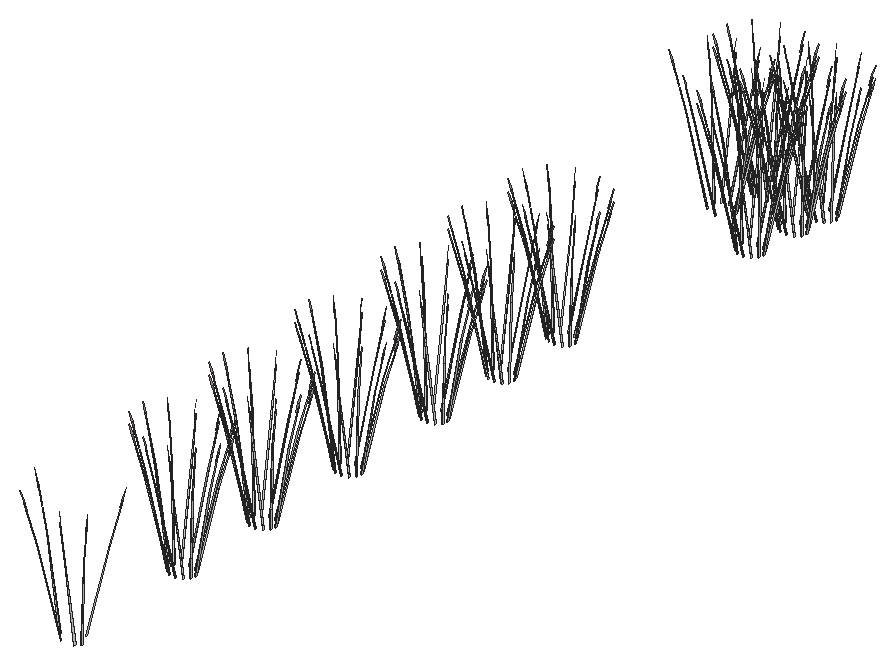
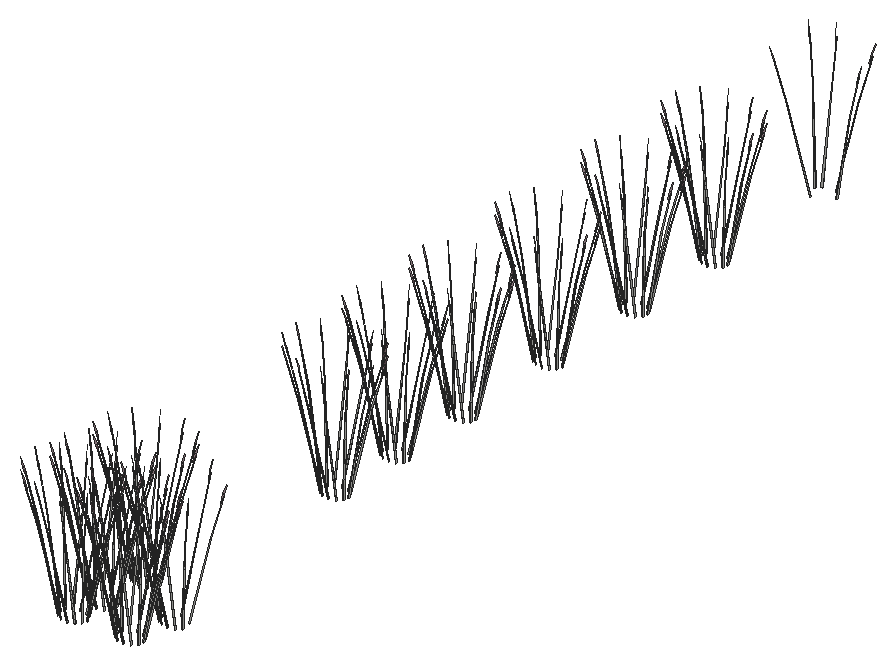
# SketchUp Ruby script. Lengths in inches.
U = 1.inch
M = Sketchup.active_model
def pt(a) = Geom::Point3d.new(a.map { |v| v * U })
def face(e, loops, mat)
  f = e.add_face(loops[0].map { |a| pt(a) })
  loops[1..].each { |l| e.add_face(l.map { |a| pt(a) }).erase! }
  f.material = f.back_material = mat if mat
  f
end
# faces: each face lists its corners as indices into pts; further lists are holes
def faces(e, pts, list, mat = nil) = list.each { |f| face(e, (f[0].is_a?(Array) ? f : [f]).map { |l| l.map { |i| pts[i] } }, mat) }
# xy, xz, yz: faces in a plane at the given z, y or x. An outline is a flat list of corners, or four numbers for a rectangle; further outlines are holes
def ring(l) = l.size == 4 ? [[l[0], l[1]], [l[2], l[1]], [l[2], l[3]], [l[0], l[3]]] : l.each_slice(2).to_a
def flat(e, list, mat, &to3) = list.each { |f| face(e, (f[0].is_a?(Array) ? f : [f]).map { |l| ring(l).map { |u, v| to3.(u, v) } }, mat) }
def xy(e, z, list, mat = nil) = flat(e, list, mat) { |x, y| [x, y, z] }
def xz(e, y, list, mat = nil) = flat(e, list, mat) { |x, z| [x, y, z] }
def yz(e, x, list, mat = nil) = flat(e, list, mat) { |y, z| [x, y, z] }
def lines(e, pts, list) = list.each { |a, b| e.add_line(pt(pts[a]), pt(pts[b])) }
# prism: a flat outline (further loops are holes) pulled along v
def prism(e, loops, v, mat = nil)
  f = face(e, loops, mat); d = Geom::Vector3d.new(v.map { |x| x * U })
  f.pushpull(f.normal.samedirection?(d) ? d.length : -d.length)
end
def box(e, o, s, mat = nil) = prism(e, [[o, [o[0] + s[0], o[1], o[2]], [o[0] + s[0], o[1] + s[1], o[2]], [o[0], o[1] + s[1], o[2]]]], [0, 0, s[2]], mat)
def at(x, y, z, deg = 0) = Geom::Transformation.translation(pt([x, y, z])) * Geom::Transformation.rotation(ORIGIN, Z_AXIS, deg.degrees)
def axes(o, x, y, z) = Geom::Transformation.new([*x, 0, *y, 0, *z, 0, *pt(o).to_a, 1])
def part(name) = M.definitions.add(name)
# library, detail: a bought-in or finely detailed component or shape, given as its bounding box
def library(name, o, s) = part(name).tap { |d| box(d.entities, o, s) }
def detail(e, o, s) = box(e.add_group.entities, o, s)
def put(e, d, t, mat = nil) = e.add_instance(d, t).tap { |i| i.material = mat if mat }
def group(e, t, mat = nil) = e.add_group.tap { |g| g.transformation = t; g.material = mat if mat }.entities
root = M.entities
M.materials.add("LightPink_Translucent").color = [144, 107, 117]
M.materials["LightPink_Translucent"].alpha = 0.75
c1 = part("blade")
p = [[2.15,0.21,22],[0,0.17,0],[0.09,0.45,0],[2.18,0.31,22],[2.29,0.31,22],[0.38,0.45,0],
  [2.48,0.24,33],[2.49,0.24,33],[2.48,0.22,33]]
faces(c1.entities,p,[[0,1,2,3],[4,5,2,3],[6,3,4,7],[8,0,3,6]])
c2 = part("seeds")
p = [[0.3,-0.1,1.38],[-0.01,-0.03,1.59],[-0.01,-0.03,0.03],[0.14,-0.07,-0.07],[0.29,-0.03,3],[0.15,0.01,3.11]]
faces(c2.entities,p,[[0,1,2,3],[1,0,4,5]],"LightPink_Translucent")
c3 = part("blade with seeds")
put(c3.entities,c1,at(0,0,0))
put(c3.entities,c2,axes([2.4,0.25,30.99],[1.5799,-0.05474,1.17369],[-0.12525,1.92788,0.29478],[-0.07173,-0.02425,1.56792]))
put(root,c3,axes([672.56,170.6875,514.19],[-0.10048,-0.4599,0.29394],[0.5744,-0.12144,-0.37948],[0.15428,0.13179,0.72609]))
put(root,c3,axes([674.22,167.95,514.19],[-0.56631,0.0816,0.29394],[-0.14954,-0.46647,-0.37948],[0.16229,-0.12529,0.72609]))
put(root,c3,axes([669.09,168.22,514.19],[0.54068,0.15928,0.29394],[-0.1577,0.46469,-0.37948],[-0.21769,0.04261,0.72609]))
put(root,c3,axes([673.45,167.02,514.19],[-0.4402,0.30062,0.29394],[-0.41671,-0.34326,-0.37948],[0.0634,-0.1744,0.72609]))
put(root,c3,axes([670.85,166.6,514.19],[0.10048,0.4599,0.29394],[-0.5744,0.12144,-0.37948],[-0.15428,-0.13179,0.72609]))
put(root,c3,axes([671.18,198.22,514.19],[0.19614,-0.43908,0.29394],[0.57222,0.12807,-0.37948],[0.05247,0.17678,0.72609]))
put(root,c3,axes([672.22,193.98,514.19],[-0.19614,0.43908,0.29394],[-0.57222,-0.12807,-0.37948],[-0.05247,-0.17678,0.72609]))
put(root,c3,axes([673.7,197.52,514.19],[-0.37017,-0.35748,0.29394],[0.42268,-0.3384,-0.37948],[0.21476,0.05149,0.72609]))
put(root,c3,axes([674.31,196.52,514.19],[-0.54068,-0.15928,0.29394],[0.1577,-0.46469,-0.37948],[0.21769,-0.04261,0.72609]))
put(root,c3,axes([669.7,194.67,514.19],[0.37017,0.35748,0.29394],[-0.42268,0.3384,-0.37948],[-0.21476,-0.05149,0.72609]))
put(root,c3,axes([669.95,197.72,514.19],[0.4402,-0.30062,0.29394],[0.41671,0.34326,-0.37948],[-0.0634,0.1744,0.72609]))
put(root,c3,axes([669.18,196.79,514.19],[0.56631,-0.0816,0.29394],[0.14954,0.46647,-0.37948],[-0.16229,0.12529,0.72609]))
put(root,c3,axes([672.56,198.14,514.19],[-0.10048,-0.4599,0.29394],[0.5744,-0.12144,-0.37948],[0.15428,0.13179,0.72609]))
put(root,c3,axes([674.22,195.4,514.19],[-0.56631,0.0816,0.29394],[-0.14954,-0.46647,-0.37948],[0.16229,-0.12529,0.72609]))
put(root,c3,axes([669.09,195.68,514.19],[0.54068,0.15928,0.29394],[-0.1577,0.46469,-0.37948],[-0.21769,0.04261,0.72609]))
put(root,c3,axes([673.45,194.48,514.19],[-0.4402,0.30062,0.29394],[-0.41671,-0.34326,-0.37948],[0.0634,-0.1744,0.72609]))
put(root,c3,axes([670.85,194.05,514.19],[0.10048,0.4599,0.29394],[-0.5744,0.12144,-0.37948],[-0.15428,-0.13179,0.72609]))
put(root,c3,axes([671.18,218.51,514.19],[0.19614,-0.43908,0.29394],[0.57222,0.12807,-0.37948],[0.05247,0.17678,0.72609]))
put(root,c3,axes([672.22,214.27,514.19],[-0.19614,0.43908,0.29394],[-0.57222,-0.12807,-0.37948],[-0.05247,-0.17678,0.72609]))
put(root,c3,axes([673.7,217.81,514.19],[-0.37017,-0.35748,0.29394],[0.42268,-0.3384,-0.37948],[0.21476,0.05149,0.72609]))
put(root,c3,axes([674.31,216.8125,514.19],[-0.54068,-0.15928,0.29394],[0.1577,-0.46469,-0.37948],[0.21769,-0.04261,0.72609]))
put(root,c3,axes([669.7,214.97,514.19],[0.37017,0.35748,0.29394],[-0.42268,0.3384,-0.37948],[-0.21476,-0.05149,0.72609]))
put(root,c3,axes([669.95,218.01,514.19],[0.4402,-0.30062,0.29394],[0.41671,0.34326,-0.37948],[-0.0634,0.1744,0.72609]))
put(root,c3,axes([669.18,217.08,514.19],[0.56631,-0.0816,0.29394],[0.14954,0.46647,-0.37948],[-0.16229,0.12529,0.72609]))
put(root,c3,axes([672.56,218.4375,514.19],[-0.10048,-0.4599,0.29394],[0.5744,-0.12144,-0.37948],[0.15428,0.13179,0.72609]))
put(root,c3,axes([674.22,215.7,514.19],[-0.56631,0.0816,0.29394],[-0.14954,-0.46647,-0.37948],[0.16229,-0.12529,0.72609]))
put(root,c3,axes([669.09,215.97,514.19],[0.54068,0.15928,0.29394],[-0.1577,0.46469,-0.37948],[-0.21769,0.04261,0.72609]))
put(root,c3,axes([673.45,214.77,514.19],[-0.4402,0.30062,0.29394],[-0.41671,-0.34326,-0.37948],[0.0634,-0.1744,0.72609]))
put(root,c3,axes([670.85,214.35,514.19],[0.10048,0.4599,0.29394],[-0.5744,0.12144,-0.37948],[-0.15428,-0.13179,0.72609]))
put(root,c3,axes([671.18,240.21,514.19],[0.19614,-0.43908,0.29394],[0.57222,0.12807,-0.37948],[0.05247,0.17678,0.72609]))
put(root,c3,axes([672.22,235.97,514.19],[-0.19614,0.43908,0.29394],[-0.57222,-0.12807,-0.37948],[-0.05247,-0.17678,0.72609]))
put(root,c3,axes([673.7,239.51,514.19],[-0.37017,-0.35748,0.29394],[0.42268,-0.3384,-0.37948],[0.21476,0.05149,0.72609]))
put(root,c3,axes([674.31,238.51,514.19],[-0.54068,-0.15928,0.29394],[0.1577,-0.46469,-0.37948],[0.21769,-0.04261,0.72609]))
put(root,c3,axes([669.7,236.66,514.19],[0.37017,0.35748,0.29394],[-0.42268,0.3384,-0.37948],[-0.21476,-0.05149,0.72609]))
put(root,c3,axes([669.95,239.71,514.19],[0.4402,-0.30062,0.29394],[0.41671,0.34326,-0.37948],[-0.0634,0.1744,0.72609]))
put(root,c3,axes([669.18,238.78,514.19],[0.56631,-0.0816,0.29394],[0.14954,0.46647,-0.37948],[-0.16229,0.12529,0.72609]))
put(root,c3,axes([672.56,240.13,514.19],[-0.10048,-0.4599,0.29394],[0.5744,-0.12144,-0.37948],[0.15428,0.13179,0.72609]))
put(root,c3,axes([674.22,237.39,514.19],[-0.56631,0.0816,0.29394],[-0.14954,-0.46647,-0.37948],[0.16229,-0.12529,0.72609]))
put(root,c3,axes([669.09,237.67,514.19],[0.54068,0.15928,0.29394],[-0.1577,0.46469,-0.37948],[-0.21769,0.04261,0.72609]))
put(root,c3,axes([673.45,236.46,514.19],[-0.4402,0.30062,0.29394],[-0.41671,-0.34326,-0.37948],[0.0634,-0.1744,0.72609]))
put(root,c3,axes([670.85,236.04,514.19],[0.10048,0.4599,0.29394],[-0.5744,0.12144,-0.37948],[-0.15428,-0.13179,0.72609]))
put(root,c3,axes([671.18,262.05,514.19],[0.19614,-0.43908,0.29394],[0.57222,0.12807,-0.37948],[0.05247,0.17678,0.72609]))
put(root,c3,axes([672.22,257.82,514.19],[-0.19614,0.43908,0.29394],[-0.57222,-0.12807,-0.37948],[-0.05247,-0.17678,0.72609]))
put(root,c3,axes([673.7,261.36,514.19],[-0.37017,-0.35748,0.29394],[0.42268,-0.3384,-0.37948],[0.21476,0.05149,0.72609]))
put(root,c3,axes([674.31,260.35,514.19],[-0.54068,-0.15928,0.29394],[0.1577,-0.46469,-0.37948],[0.21769,-0.04261,0.72609]))
put(root,c3,axes([669.7,258.51,514.19],[0.37017,0.35748,0.29394],[-0.42268,0.3384,-0.37948],[-0.21476,-0.05149,0.72609]))
put(root,c3,axes([669.95,261.56,514.19],[0.4402,-0.30062,0.29394],[0.41671,0.34326,-0.37948],[-0.0634,0.1744,0.72609]))
put(root,c3,axes([669.18,260.63,514.19],[0.56631,-0.0816,0.29394],[0.14954,0.46647,-0.37948],[-0.16229,0.12529,0.72609]))
put(root,c3,axes([672.56,261.98,514.19],[-0.10048,-0.4599,0.29394],[0.5744,-0.12144,-0.37948],[0.15428,0.13179,0.72609]))
put(root,c3,axes([674.22,259.24,514.19],[-0.56631,0.0816,0.29394],[-0.14954,-0.46647,-0.37948],[0.16229,-0.12529,0.72609]))
put(root,c3,axes([669.09,259.51,514.19],[0.54068,0.15928,0.29394],[-0.1577,0.46469,-0.37948],[-0.21769,0.04261,0.72609]))
put(root,c3,axes([673.45,258.31,514.19],[-0.4402,0.30062,0.29394],[-0.41671,-0.34326,-0.37948],[0.0634,-0.1744,0.72609]))
put(root,c3,axes([670.85,257.89,514.19],[0.10048,0.4599,0.29394],[-0.5744,0.12144,-0.37948],[-0.15428,-0.13179,0.72609]))
put(root,c3,axes([671.18,278.91,514.19],[0.19614,-0.43908,0.29394],[0.57222,0.12807,-0.37948],[0.05247,0.17678,0.72609]))
put(root,c3,axes([672.22,274.67,514.19],[-0.19614,0.43908,0.29394],[-0.57222,-0.12807,-0.37948],[-0.05247,-0.17678,0.72609]))
put(root,c3,axes([673.7,278.22,514.19],[-0.37017,-0.35748,0.29394],[0.42268,-0.3384,-0.37948],[0.21476,0.05149,0.72609]))
put(root,c3,axes([674.31,277.21,514.19],[-0.54068,-0.15928,0.29394],[0.1577,-0.46469,-0.37948],[0.21769,-0.04261,0.72609]))
put(root,c3,axes([669.7,275.37,514.19],[0.37017,0.35748,0.29394],[-0.42268,0.3384,-0.37948],[-0.21476,-0.05149,0.72609]))
put(root,c3,axes([669.95,278.42,514.19],[0.4402,-0.30062,0.29394],[0.41671,0.34326,-0.37948],[-0.0634,0.1744,0.72609]))
put(root,c3,axes([669.18,277.49,514.19],[0.56631,-0.0816,0.29394],[0.14954,0.46647,-0.37948],[-0.16229,0.12529,0.72609]))
put(root,c3,axes([672.56,278.84,514.19],[-0.10048,-0.4599,0.29394],[0.5744,-0.12144,-0.37948],[0.15428,0.13179,0.72609]))
put(root,c3,axes([674.22,276.1,514.19],[-0.56631,0.0816,0.29394],[-0.14954,-0.46647,-0.37948],[0.16229,-0.12529,0.72609]))
put(root,c3,axes([669.09,276.37,514.19],[0.54068,0.15928,0.29394],[-0.1577,0.46469,-0.37948],[-0.21769,0.04261,0.72609]))
put(root,c3,axes([673.45,275.17,514.19],[-0.4402,0.30062,0.29394],[-0.41671,-0.34326,-0.37948],[0.0634,-0.1744,0.72609]))
put(root,c3,axes([670.85,274.75,514.19],[0.10048,0.4599,0.29394],[-0.5744,0.12144,-0.37948],[-0.15428,-0.13179,0.72609]))
put(root,c3,axes([671.18,294.24,514.19],[0.19614,-0.43908,0.29394],[0.57222,0.12807,-0.37948],[0.05247,0.17678,0.72609]))
put(root,c3,axes([672.22,290.01,514.19],[-0.19614,0.43908,0.29394],[-0.57222,-0.12807,-0.37948],[-0.05247,-0.17678,0.72609]))
put(root,c3,axes([673.7,293.55,514.19],[-0.37017,-0.35748,0.29394],[0.42268,-0.3384,-0.37948],[0.21476,0.05149,0.72609]))
put(root,c3,axes([674.31,292.55,514.19],[-0.54068,-0.15928,0.29394],[0.1577,-0.46469,-0.37948],[0.21769,-0.04261,0.72609]))
put(root,c3,axes([669.7,290.7,514.19],[0.37017,0.35748,0.29394],[-0.42268,0.3384,-0.37948],[-0.21476,-0.05149,0.72609]))
put(root,c3,axes([669.95,293.75,514.19],[0.4402,-0.30062,0.29394],[0.41671,0.34326,-0.37948],[-0.0634,0.1744,0.72609]))
put(root,c3,axes([669.18,292.82,514.19],[0.56631,-0.0816,0.29394],[0.14954,0.46647,-0.37948],[-0.16229,0.12529,0.72609]))
put(root,c3,axes([672.56,294.17,514.19],[-0.10048,-0.4599,0.29394],[0.5744,-0.12144,-0.37948],[0.15428,0.13179,0.72609]))
put(root,c3,axes([674.22,291.43,514.19],[-0.56631,0.0816,0.29394],[-0.14954,-0.46647,-0.37948],[0.16229,-0.12529,0.72609]))
put(root,c3,axes([669.09,291.71,514.19],[0.54068,0.15928,0.29394],[-0.1577,0.46469,-0.37948],[-0.21769,0.04261,0.72609]))
put(root,c3,axes([673.45,290.5,514.19],[-0.4402,0.30062,0.29394],[-0.41671,-0.34326,-0.37948],[0.0634,-0.1744,0.72609]))
put(root,c3,axes([670.85,290.08,514.19],[0.10048,0.4599,0.29394],[-0.5744,0.12144,-0.37948],[-0.15428,-0.13179,0.72609]))
put(root,c3,axes([678.57,351.17,514.19],[0.19614,-0.43908,0.29394],[0.57222,0.12807,-0.37948],[0.05247,0.17678,0.72609]))
put(root,c3,axes([679.6,346.93,514.19],[-0.19614,0.43908,0.29394],[-0.57222,-0.12807,-0.37948],[-0.05247,-0.17678,0.72609]))
put(root,c3,axes([681.08,350.47,514.19],[-0.37017,-0.35748,0.29394],[0.42268,-0.3384,-0.37948],[0.21476,0.05149,0.72609]))
put(root,c3,axes([681.69,349.47,514.19],[-0.54068,-0.15928,0.29394],[0.1577,-0.46469,-0.37948],[0.21769,-0.04261,0.72609]))
put(root,c3,axes([677.09,347.625,514.19],[0.37017,0.35748,0.29394],[-0.42268,0.3384,-0.37948],[-0.21476,-0.05149,0.72609]))
put(root,c3,axes([677.33,350.67,514.19],[0.4402,-0.30062,0.29394],[0.41671,0.34326,-0.37948],[-0.0634,0.1744,0.72609]))
put(root,c3,axes([676.57,349.74,514.19],[0.56631,-0.0816,0.29394],[0.14954,0.46647,-0.37948],[-0.16229,0.12529,0.72609]))
put(root,c3,axes([679.94,351.1,514.19],[-0.10048,-0.4599,0.29394],[0.5744,-0.12144,-0.37948],[0.15428,0.13179,0.72609]))
put(root,c3,axes([681.6,348.36,514.19],[-0.56631,0.0816,0.29394],[-0.14954,-0.46647,-0.37948],[0.16229,-0.12529,0.72609]))
put(root,c3,axes([676.48,348.63,514.19],[0.54068,0.15928,0.29394],[-0.1577,0.46469,-0.37948],[-0.21769,0.04261,0.72609]))
put(root,c3,axes([680.84,347.43,514.19],[-0.4402,0.30062,0.29394],[-0.41671,-0.34326,-0.37948],[0.0634,-0.1744,0.72609]))
put(root,c3,axes([678.23,347.01,514.19],[0.10048,0.4599,0.29394],[-0.5744,0.12144,-0.37948],[-0.15428,-0.13179,0.72609]))
put(root,c3,axes([677.62,344.84,514.19],[0.19614,-0.43908,0.29394],[0.57222,0.12807,-0.37948],[0.05247,0.17678,0.72609]))
put(root,c3,axes([678.65,340.6,514.19],[-0.19614,0.43908,0.29394],[-0.57222,-0.12807,-0.37948],[-0.05247,-0.17678,0.72609]))
put(root,c3,axes([680.13,344.14,514.19],[-0.37017,-0.35748,0.29394],[0.42268,-0.3384,-0.37948],[0.21476,0.05149,0.72609]))
put(root,c3,axes([680.74,343.14,514.19],[-0.54068,-0.15928,0.29394],[0.1577,-0.46469,-0.37948],[0.21769,-0.04261,0.72609]))
put(root,c3,axes([676.14,341.29,514.19],[0.37017,0.35748,0.29394],[-0.42268,0.3384,-0.37948],[-0.21476,-0.05149,0.72609]))
put(root,c3,axes([676.38,344.34,514.19],[0.4402,-0.30062,0.29394],[0.41671,0.34326,-0.37948],[-0.0634,0.1744,0.72609]))
put(root,c3,axes([675.62,343.41,514.19],[0.56631,-0.0816,0.29394],[0.14954,0.46647,-0.37948],[-0.16229,0.12529,0.72609]))
put(root,c3,axes([678.99,344.76,514.19],[-0.10048,-0.4599,0.29394],[0.5744,-0.12144,-0.37948],[0.15428,0.13179,0.72609]))
put(root,c3,axes([680.65,342.02,514.19],[-0.56631,0.0816,0.29394],[-0.14954,-0.46647,-0.37948],[0.16229,-0.12529,0.72609]))
put(root,c3,axes([675.53,342.3,514.19],[0.54068,0.15928,0.29394],[-0.1577,0.46469,-0.37948],[-0.21769,0.04261,0.72609]))
put(root,c3,axes([679.89,341.1,514.19],[-0.4402,0.30062,0.29394],[-0.41671,-0.34326,-0.37948],[0.0634,-0.1744,0.72609]))
put(root,c3,axes([677.28,340.67,514.19],[0.10048,0.4599,0.29394],[-0.5744,0.12144,-0.37948],[-0.15428,-0.13179,0.72609]))
put(root,c3,axes([676.63,335.16,514.19],[0.19614,-0.43908,0.29394],[0.57222,0.12807,-0.37948],[0.05247,0.17678,0.72609]))
put(root,c3,axes([677.67,330.92,514.19],[-0.19614,0.43908,0.29394],[-0.57222,-0.12807,-0.37948],[-0.05247,-0.17678,0.72609]))
put(root,c3,axes([679.15,334.47,514.19],[-0.37017,-0.35748,0.29394],[0.42268,-0.3384,-0.37948],[0.21476,0.05149,0.72609]))
put(root,c3,axes([679.75,333.46,514.19],[-0.54068,-0.15928,0.29394],[0.1577,-0.46469,-0.37948],[0.21769,-0.04261,0.72609]))
put(root,c3,axes([675.15,331.62,514.19],[0.37017,0.35748,0.29394],[-0.42268,0.3384,-0.37948],[-0.21476,-0.05149,0.72609]))
put(root,c3,axes([675.39,334.67,514.19],[0.4402,-0.30062,0.29394],[0.41671,0.34326,-0.37948],[-0.0634,0.1744,0.72609]))
put(root,c3,axes([674.63,333.74,514.19],[0.56631,-0.0816,0.29394],[0.14954,0.46647,-0.37948],[-0.16229,0.12529,0.72609]))
put(root,c3,axes([678,335.09,514.19],[-0.10048,-0.4599,0.29394],[0.5744,-0.12144,-0.37948],[0.15428,0.13179,0.72609]))
put(root,c3,axes([679.66,332.35,514.19],[-0.56631,0.0816,0.29394],[-0.14954,-0.46647,-0.37948],[0.16229,-0.12529,0.72609]))
put(root,c3,axes([674.54,332.62,514.19],[0.54068,0.15928,0.29394],[-0.1577,0.46469,-0.37948],[-0.21769,0.04261,0.72609]))
put(root,c3,axes([678.9,331.42,514.19],[-0.4402,0.30062,0.29394],[-0.41671,-0.34326,-0.37948],[0.0634,-0.1744,0.72609]))
put(root,c3,axes([676.29,331,514.19],[0.10048,0.4599,0.29394],[-0.5744,0.12144,-0.37948],[-0.15428,-0.13179,0.72609]))
put(root,c3,axes([667.26,350.97,514.19],[0.19614,-0.43908,0.29394],[0.57222,0.12807,-0.37948],[0.05247,0.17678,0.72609]))
put(root,c3,axes([668.3,346.73,514.19],[-0.19614,0.43908,0.29394],[-0.57222,-0.12807,-0.37948],[-0.05247,-0.17678,0.72609]))
put(root,c3,axes([669.78,350.27,514.19],[-0.37017,-0.35748,0.29394],[0.42268,-0.3384,-0.37948],[0.21476,0.05149,0.72609]))
put(root,c3,axes([670.39,349.27,514.19],[-0.54068,-0.15928,0.29394],[0.1577,-0.46469,-0.37948],[0.21769,-0.04261,0.72609]))
put(root,c3,axes([665.78,347.42,514.19],[0.37017,0.35748,0.29394],[-0.42268,0.3384,-0.37948],[-0.21476,-0.05149,0.72609]))
put(root,c3,axes([666.02,350.47,514.19],[0.4402,-0.30062,0.29394],[0.41671,0.34326,-0.37948],[-0.0634,0.1744,0.72609]))
put(root,c3,axes([665.26,349.54,514.19],[0.56631,-0.0816,0.29394],[0.14954,0.46647,-0.37948],[-0.16229,0.12529,0.72609]))
put(root,c3,axes([668.63,350.89,514.19],[-0.10048,-0.4599,0.29394],[0.5744,-0.12144,-0.37948],[0.15428,0.13179,0.72609]))
put(root,c3,axes([670.3,348.15,514.19],[-0.56631,0.0816,0.29394],[-0.14954,-0.46647,-0.37948],[0.16229,-0.12529,0.72609]))
put(root,c3,axes([665.17,348.43,514.19],[0.54068,0.15928,0.29394],[-0.1577,0.46469,-0.37948],[-0.21769,0.04261,0.72609]))
put(root,c3,axes([669.53,347.22,514.19],[-0.4402,0.30062,0.29394],[-0.41671,-0.34326,-0.37948],[0.0634,-0.1744,0.72609]))
put(root,c3,axes([666.92,346.8,514.19],[0.10048,0.4599,0.29394],[-0.5744,0.12144,-0.37948],[-0.15428,-0.13179,0.72609]))
put(root,c3,axes([665,342.625,514.19],[0.19614,-0.43908,0.29394],[0.57222,0.12807,-0.37948],[0.05247,0.17678,0.72609]))
put(root,c3,axes([666.04,338.39,514.19],[-0.19614,0.43908,0.29394],[-0.57222,-0.12807,-0.37948],[-0.05247,-0.17678,0.72609]))
put(root,c3,axes([667.52,341.93,514.19],[-0.37017,-0.35748,0.29394],[0.42268,-0.3384,-0.37948],[0.21476,0.05149,0.72609]))
put(root,c3,axes([668.13,340.93,514.19],[-0.54068,-0.15928,0.29394],[0.1577,-0.46469,-0.37948],[0.21769,-0.04261,0.72609]))
put(root,c3,axes([663.52,339.08,514.19],[0.37017,0.35748,0.29394],[-0.42268,0.3384,-0.37948],[-0.21476,-0.05149,0.72609]))
put(root,c3,axes([663.77,342.13,514.19],[0.4402,-0.30062,0.29394],[0.41671,0.34326,-0.37948],[-0.0634,0.1744,0.72609]))
put(root,c3,axes([663,341.2,514.19],[0.56631,-0.0816,0.29394],[0.14954,0.46647,-0.37948],[-0.16229,0.12529,0.72609]))
put(root,c3,axes([666.375,342.55,514.19],[-0.10048,-0.4599,0.29394],[0.5744,-0.12144,-0.37948],[0.15428,0.13179,0.72609]))
